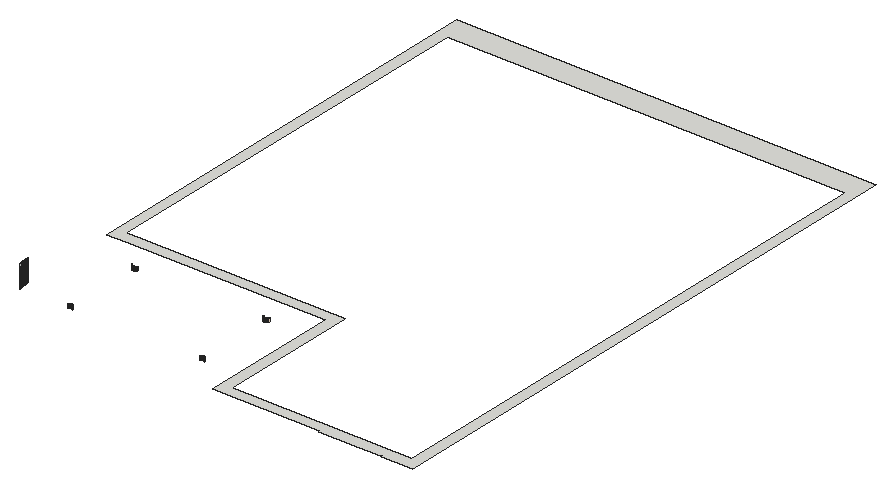
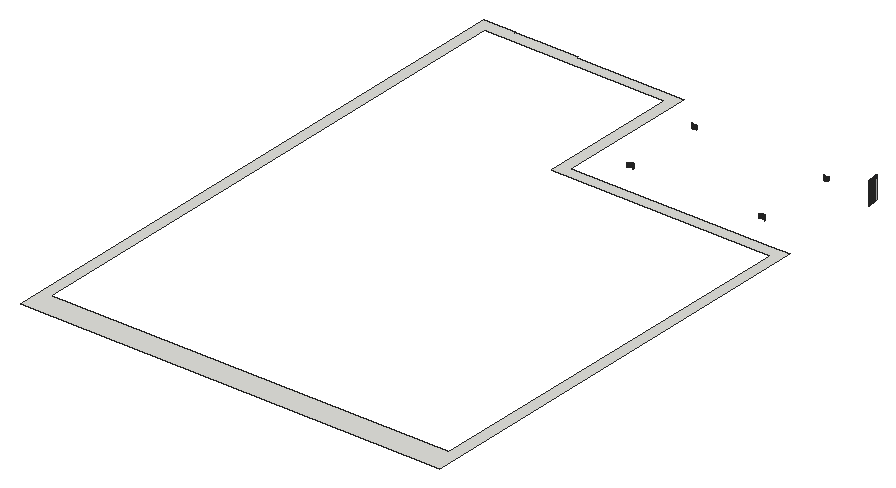
# SketchUp Ruby script. Lengths in inches.
U = 1.inch
M = Sketchup.active_model
def pt(a) = Geom::Point3d.new(a.map { |v| v * U })
def face(e, loops, mat)
  f = e.add_face(loops[0].map { |a| pt(a) })
  loops[1..].each { |l| e.add_face(l.map { |a| pt(a) }).erase! }
  f.material = f.back_material = mat if mat
  f
end
# faces: each face lists its corners as indices into pts; further lists are holes
def faces(e, pts, list, mat = nil) = list.each { |f| face(e, (f[0].is_a?(Array) ? f : [f]).map { |l| l.map { |i| pts[i] } }, mat) }
# xy, xz, yz: faces in a plane at the given z, y or x. An outline is a flat list of corners, or four numbers for a rectangle; further outlines are holes
def ring(l) = l.size == 4 ? [[l[0], l[1]], [l[2], l[1]], [l[2], l[3]], [l[0], l[3]]] : l.each_slice(2).to_a
def flat(e, list, mat, &to3) = list.each { |f| face(e, (f[0].is_a?(Array) ? f : [f]).map { |l| ring(l).map { |u, v| to3.(u, v) } }, mat) }
def xy(e, z, list, mat = nil) = flat(e, list, mat) { |x, y| [x, y, z] }
def xz(e, y, list, mat = nil) = flat(e, list, mat) { |x, z| [x, y, z] }
def yz(e, x, list, mat = nil) = flat(e, list, mat) { |y, z| [x, y, z] }
def lines(e, pts, list) = list.each { |a, b| e.add_line(pt(pts[a]), pt(pts[b])) }
# prism: a flat outline (further loops are holes) pulled along v
def prism(e, loops, v, mat = nil)
  f = face(e, loops, mat); d = Geom::Vector3d.new(v.map { |x| x * U })
  f.pushpull(f.normal.samedirection?(d) ? d.length : -d.length)
end
def box(e, o, s, mat = nil) = prism(e, [[o, [o[0] + s[0], o[1], o[2]], [o[0] + s[0], o[1] + s[1], o[2]], [o[0], o[1] + s[1], o[2]]]], [0, 0, s[2]], mat)
def at(x, y, z, deg = 0) = Geom::Transformation.translation(pt([x, y, z])) * Geom::Transformation.rotation(ORIGIN, Z_AXIS, deg.degrees)
def axes(o, x, y, z) = Geom::Transformation.new([*x, 0, *y, 0, *z, 0, *pt(o).to_a, 1])
def part(name) = M.definitions.add(name)
# library, detail: a bought-in or finely detailed component or shape, given as its bounding box
def library(name, o, s) = part(name).tap { |d| box(d.entities, o, s) }
def detail(e, o, s) = box(e.add_group.entities, o, s)
def put(e, d, t, mat = nil) = e.add_instance(d, t).tap { |i| i.material = mat if mat }
def group(e, t, mat = nil) = e.add_group.tap { |g| g.transformation = t; g.material = mat if mat }.entities
root = M.entities
M.materials.add("1122 AP 7994 PEACH ROSE").color = [254, 227, 201]
M.materials.add("[Quartz Light Grey]").color = [251, 251, 252]
xy(root,278.82,[[[286.125,152,320.75,152,320.75,153.25,321,153.25,321,152,338.75,152,338.75,153.25,339.75,153.25,339.75,152,366,152,366,645,9,645,9,273,25,273,25,273.25,25.25,273.25,25.25,273,195,273,195,153,286.125,153],[204,162,204,282,18,282,18,624,357,624,357,162]]])
xz(root,180,[[52.82,278.82,52.9,281.82],[52.9,278.82,52.98,281.82],[52.98,278.82,53.06,281.82],[53.06,278.82,53.14,281.82],[164.84,278.82,164.92,281.82],
  [164.92,278.82,165,281.82],[165,278.82,165.08,281.82],[165.08,278.82,165.16,281.82]],"1122 AP 7994 PEACH ROSE")
xz(root,246,[[52.82,278.82,52.9,281.82],[52.9,278.82,52.98,281.82],[52.98,278.82,53.06,281.82],[53.06,278.82,53.14,281.82],[164.84,278.82,164.92,281.82],
  [164.92,278.82,165,281.82],[165,278.82,165.08,281.82],[165.08,278.82,165.16,281.82]],"1122 AP 7994 PEACH ROSE")
yz(root,9,[[188.6875,278.82,189,297.82]],"[Quartz Light Grey]")
yz(root,9.01,[[188.06,278.82,188.37,297.82]],"[Quartz Light Grey]")
p = [[50.75,179.01,278.82],[50.8,179.07,278.82],[50.8,179.07,281.82],[50.75,179.01,281.82],[55.16,179.07,278.82],[55.21,179.01,278.82],
  [55.21,179.01,281.82],[55.16,179.07,281.82],[162.77,179.01,278.82],[162.82,179.07,278.82],[162.82,179.07,281.82],[162.77,179.01,281.82],
  [167.18,179.07,278.82],[167.23,179.01,278.82],[167.23,179.01,281.82],[167.18,179.07,281.82],[10.31,179.38,278.82],[10.39,179.08,278.82],
  [10.39,179.08,297.82],[10.31,179.38,297.82],[50.86,179.12,278.82],[50.86,179.12,281.82],[50.92,179.18,278.82],[50.92,179.18,281.82],
  [55.05,179.18,278.82],[55.1,179.12,278.82],[55.1,179.12,281.82],[55.05,179.18,281.82],[162.88,179.12,278.82],[162.88,179.12,281.82],
  [162.93,179.18,278.82],[162.93,179.18,281.82],[167.12,179.12,278.82],[167.12,179.12,281.82],[167.07,179.18,278.82],[167.07,179.18,281.82],
  [50.97,179.23,278.82],[50.97,179.23,281.82],[51.03,179.28,278.82],[51.03,179.28,281.82],[54.93,179.28,278.82],[54.99,179.23,278.82],
  [54.99,179.23,281.82],[54.93,179.28,281.82],[162.99,179.23,278.82],[162.99,179.23,281.82],[163.05,179.28,278.82],[163.05,179.28,281.82],
  [166.95,179.28,278.82],[167.01,179.23,278.82],[167.01,179.23,281.82],[166.95,179.28,281.82],[51.09,179.33,278.82],[51.09,179.33,281.82],
  [51.15,179.38,278.82],[51.15,179.38,281.82],[54.81,179.38,278.82],[54.87,179.33,278.82],[54.87,179.33,281.82],[54.81,179.38,281.82],
  [163.11,179.33,278.82],[163.11,179.33,281.82],[163.17,179.38,278.82],[163.17,179.38,281.82],[166.83,179.38,278.82],[166.89,179.33,278.82],
  [166.89,179.33,281.82],[166.83,179.38,281.82],[10.23,179.68,278.82],[10.23,179.68,297.82],[51.22,179.43,278.82],[51.22,179.43,281.82],
  [51.28,179.47,278.82],[51.28,179.47,281.82],[54.74,179.43,278.82],[54.74,179.43,281.82],[54.68,179.47,278.82],[54.68,179.47,281.82],
  [163.24,179.43,278.82],[163.24,179.43,281.82],[163.3,179.47,278.82],[163.3,179.47,281.82],[166.7,179.47,278.82],[166.76,179.43,278.82],
  [166.76,179.43,281.82],[166.7,179.47,281.82],[51.35,179.52,278.82],[51.35,179.52,281.82],[51.41,179.56,278.82],[51.41,179.56,281.82],
  [54.55,179.56,278.82],[54.61,179.52,278.82],[54.61,179.52,281.82],[54.55,179.56,281.82],[163.37,179.52,278.82],[163.37,179.52,281.82],
  [163.43,179.56,278.82],[163.43,179.56,281.82],[166.63,179.52,278.82],[166.63,179.52,281.82],[166.57,179.56,278.82],[166.57,179.56,281.82],
  [51.48,179.6,278.82],[51.48,179.6,281.82],[51.55,179.64,278.82],[51.55,179.64,281.82],[51.62,179.67,278.82],[51.62,179.67,281.82],
  [54.34,179.67,278.82],[54.41,179.64,278.82],[54.41,179.64,281.82],[54.34,179.67,281.82],[54.48,179.6,278.82],[54.48,179.6,281.82],
  [163.5,179.6,278.82],[163.5,179.6,281.82],[163.57,179.64,278.82],[163.57,179.64,281.82],[163.64,179.67,278.82],[163.64,179.67,281.82],
  [166.43,179.64,278.82],[166.5,179.6,278.82],[166.5,179.6,281.82],[166.43,179.64,281.82],[166.36,179.67,278.82],[166.36,179.67,281.82],
  [10.15,179.99,278.82],[10.15,179.99,297.82],[51.6875,179.71,278.82],[51.6875,179.71,281.82],[51.76,179.74,278.82],[51.76,179.74,281.82],
  [51.83,179.77,278.82],[51.83,179.77,281.82],[54.13,179.77,278.82],[54.2,179.74,278.82],[54.2,179.74,281.82],[54.13,179.77,281.82],
  [54.27,179.71,278.82],[54.27,179.71,281.82],[163.71,179.71,278.82],[163.71,179.71,281.82],[163.78,179.74,278.82],[163.78,179.74,281.82],
  [163.85,179.77,278.82],[163.85,179.77,281.82],[166.15,179.77,278.82],[166.22,179.74,278.82],[166.22,179.74,281.82],[166.15,179.77,281.82],
  [166.29,179.71,278.82],[166.29,179.71,281.82],[51.91,179.8,278.82],[51.91,179.8,281.82],[51.98,179.83,278.82],[51.98,179.83,281.82],
  [52.05,179.85,278.82],[52.05,179.85,281.82],[53.91,179.85,278.82],[53.98,179.83,278.82],[53.98,179.83,281.82],[53.91,179.85,281.82],
  [54.06,179.8,278.82],[54.06,179.8,281.82],[163.92,179.8,278.82],[163.92,179.8,281.82],[164,179.83,278.82],[164,179.83,281.82],
  [164.07,179.85,278.82],[164.07,179.85,281.82],[165.93,179.85,278.82],[166,179.83,278.82],[166,179.83,281.82],[165.93,179.85,281.82],
  [166.08,179.8,278.82],[166.08,179.8,281.82],[52.13,179.875,278.82],[52.13,179.875,281.82],[52.2,179.9,278.82],[52.2,179.9,281.82],
  [52.28,179.92,278.82],[52.28,179.92,281.82],[52.36,179.93,278.82],[52.36,179.93,281.82],[52.43,179.95,278.82],[52.43,179.95,281.82],
  [52.51,179.96,278.82],[52.51,179.96,281.82],[53.53,179.95,278.82],[53.6,179.93,278.82],[53.6,179.93,281.82],[53.53,179.95,281.82],
  [53.45,179.96,278.82],[53.45,179.96,281.82],[53.68,179.92,278.82],[53.68,179.92,281.82],[53.76,179.9,278.82],[53.76,179.9,281.82],
  [53.83,179.875,278.82],[53.83,179.875,281.82],[164.15,179.875,278.82],[164.15,179.875,281.82],[164.22,179.9,278.82],[164.22,179.9,281.82],
  [164.3,179.92,278.82],[164.3,179.92,281.82],[164.375,179.93,278.82],[164.375,179.93,281.82],[164.45,179.95,278.82],[164.45,179.95,281.82],
  [164.53,179.96,278.82],[164.53,179.96,281.82],[165.55,179.95,278.82],[165.625,179.93,278.82],[165.625,179.93,281.82],[165.55,179.95,281.82],
  [165.47,179.96,278.82],[165.47,179.96,281.82],[165.7,179.92,278.82],[165.7,179.92,281.82],[165.78,179.9,278.82],[165.78,179.9,281.82],
  [165.85,179.875,278.82],[165.85,179.875,281.82],[10.07,180.29,278.82],[10.07,180.29,297.82],[52.59,179.97,278.82],[52.59,179.97,281.82],
  [52.67,179.98,278.82],[52.67,179.98,281.82],[52.75,179.99,278.82],[52.75,179.99,281.82],[52.82,180,278.82],[52.82,180,281.82],
  [53.14,180,278.82],[53.22,179.99,278.82],[53.22,179.99,281.82],[53.14,180,281.82],[53.29,179.98,278.82],[53.29,179.98,281.82],
  [53.37,179.97,278.82],[53.37,179.97,281.82],[164.61,179.97,278.82],[164.61,179.97,281.82],[164.6875,179.98,278.82],[164.6875,179.98,281.82],
  [164.76,179.99,278.82],[164.76,179.99,281.82],[164.84,180,278.82],[164.84,180,281.82],[165.24,179.99,278.82],[165.3125,179.98,278.82],
  [165.3125,179.98,281.82],[165.24,179.99,281.82],[165.16,180,278.82],[165.16,180,281.82],[165.39,179.97,278.82],[165.39,179.97,281.82],
  [9.99,180.6,278.82],[9.99,180.6,297.82],[9.92,180.9,278.82],[9.92,180.9,297.82],[9.85,181.21,278.82],[9.85,181.21,297.82],
  [9.79,181.52,278.82],[9.79,181.52,297.82],[9.72,181.82,278.82],[9.72,181.82,297.82],[9.66,182.13,278.82],[9.66,182.13,297.82],
  [9.6,182.44,278.82],[9.6,182.44,297.82],[9.55,182.75,278.82],[9.55,182.75,297.82],[9.49,183.06,278.82],[9.49,183.06,297.82],
  [9.44,183.37,278.82],[9.44,183.37,297.82],[9.4,183.68,278.82],[9.4,183.68,297.82],[9.35,183.99,278.82],[9.35,183.99,297.82],
  [9.31,184.3,278.82],[9.31,184.3,297.82],[9.27,184.61,278.82],[9.27,184.61,297.82],[9.23,184.92,278.82],[9.23,184.92,297.82],
  [9.2,185.24,278.82],[9.2,185.24,297.82],[9.17,185.55,278.82],[9.17,185.55,297.82],[9.14,185.86,278.82],[9.14,185.86,297.82],
  [9.11,186.18,278.82],[9.11,186.18,297.82],[9.09,186.49,278.82],[9.09,186.49,297.82],[9.07,186.8,278.82],[9.07,186.8,297.82],
  [9.05,187.12,278.82],[9.05,187.12,297.82],[9.03,187.43,278.82],[9.03,187.43,297.82],[9.02,187.74,278.82],[9.02,187.74,297.82],
  [9.01,188.06,278.82],[9.01,188.06,297.82],[9,188.6875,278.82],[9.01,188.37,278.82],[9.01,188.37,297.82],[9,188.6875,297.82],
  [52.51,246.04,278.82],[52.43,246.05,278.82],[52.43,246.05,281.82],[52.51,246.04,281.82],[52.59,246.03,278.82],[52.59,246.03,281.82],
  [52.67,246.02,278.82],[52.67,246.02,281.82],[52.82,246,278.82],[52.75,246.01,278.82],[52.75,246.01,281.82],[52.82,246,281.82],
  [53.22,246.01,278.82],[53.14,246,278.82],[53.14,246,281.82],[53.22,246.01,281.82],[53.29,246.02,278.82],[53.29,246.02,281.82],
  [53.37,246.03,278.82],[53.37,246.03,281.82],[53.45,246.04,278.82],[53.45,246.04,281.82],[53.53,246.05,278.82],[53.53,246.05,281.82],
  [164.61,246.03,278.82],[164.53,246.04,278.82],[164.53,246.04,281.82],[164.61,246.03,281.82],[164.45,246.05,278.82],[164.45,246.05,281.82],
  [164.6875,246.02,278.82],[164.6875,246.02,281.82],[164.76,246.01,278.82],[164.76,246.01,281.82],[164.84,246,278.82],[164.84,246,281.82],
  [165.24,246.01,278.82],[165.16,246,278.82],[165.16,246,281.82],[165.24,246.01,281.82],[165.3125,246.02,278.82],[165.3125,246.02,281.82],
  [165.39,246.03,278.82],[165.39,246.03,281.82],[165.47,246.04,278.82],[165.47,246.04,281.82],[165.55,246.05,278.82],[165.55,246.05,281.82],
  [52.05,246.15,278.82],[51.98,246.17,278.82],[51.98,246.17,281.82],[52.05,246.15,281.82],[52.2,246.1,278.82],[52.13,246.125,278.82],
  [52.13,246.125,281.82],[52.2,246.1,281.82],[52.28,246.08,278.82],[52.28,246.08,281.82],[52.36,246.07,278.82],[52.36,246.07,281.82],
  [53.6,246.07,278.82],[53.6,246.07,281.82],[53.68,246.08,278.82],[53.68,246.08,281.82],[53.76,246.1,278.82],[53.76,246.1,281.82],
  [53.83,246.125,278.82],[53.83,246.125,281.82],[53.91,246.15,278.82],[53.91,246.15,281.82],[53.98,246.17,278.82],[53.98,246.17,281.82],
  [164.07,246.15,278.82],[164,246.17,278.82],[164,246.17,281.82],[164.07,246.15,281.82],[164.22,246.1,278.82],[164.15,246.125,278.82],
  [164.15,246.125,281.82],[164.22,246.1,281.82],[164.3,246.08,278.82],[164.3,246.08,281.82],[164.375,246.07,278.82],[164.375,246.07,281.82],
  [165.625,246.07,278.82],[165.625,246.07,281.82],[165.7,246.08,278.82],[165.7,246.08,281.82],[165.78,246.1,278.82],[165.78,246.1,281.82],
  [165.85,246.125,278.82],[165.85,246.125,281.82],[165.93,246.15,278.82],[165.93,246.15,281.82],[166,246.17,278.82],[166,246.17,281.82],
  [51.91,246.2,278.82],[51.83,246.23,278.82],[51.83,246.23,281.82],[51.91,246.2,281.82],[51.76,246.26,278.82],[51.76,246.26,281.82],
  [54.06,246.2,278.82],[54.06,246.2,281.82],[54.13,246.23,278.82],[54.13,246.23,281.82],[54.2,246.26,278.82],[54.2,246.26,281.82],
  [163.85,246.23,278.82],[163.78,246.26,278.82],[163.78,246.26,281.82],[163.85,246.23,281.82],[163.92,246.2,278.82],[163.92,246.2,281.82],
  [166.08,246.2,278.82],[166.08,246.2,281.82],[166.15,246.23,278.82],[166.15,246.23,281.82],[166.22,246.26,278.82],[166.22,246.26,281.82],
  [51.62,246.33,278.82],[51.55,246.36,278.82],[51.55,246.36,281.82],[51.62,246.33,281.82],[51.6875,246.29,278.82],[51.6875,246.29,281.82],
  [54.27,246.29,278.82],[54.27,246.29,281.82],[54.34,246.33,278.82],[54.34,246.33,281.82],[54.41,246.36,278.82],[54.41,246.36,281.82],
  [163.71,246.29,278.82],[163.64,246.33,278.82],[163.64,246.33,281.82],[163.71,246.29,281.82],[163.57,246.36,278.82],[163.57,246.36,281.82],
  [166.29,246.29,278.82],[166.29,246.29,281.82],[166.36,246.33,278.82],[166.36,246.33,281.82],[166.43,246.36,278.82],[166.43,246.36,281.82],
  [51.41,246.44,278.82],[51.35,246.48,278.82],[51.35,246.48,281.82],[51.41,246.44,281.82],[51.48,246.4,278.82],[51.48,246.4,281.82],
  [54.48,246.4,278.82],[54.48,246.4,281.82],[54.55,246.44,278.82],[54.55,246.44,281.82],[54.61,246.48,278.82],[54.61,246.48,281.82],
  [163.5,246.4,278.82],[163.43,246.44,278.82],[163.43,246.44,281.82],[163.5,246.4,281.82],[163.37,246.48,278.82],[163.37,246.48,281.82],
  [166.5,246.4,278.82],[166.5,246.4,281.82],[166.57,246.44,278.82],[166.57,246.44,281.82],[166.63,246.48,278.82],[166.63,246.48,281.82],
  [51.28,246.53,278.82],[51.22,246.57,278.82],[51.22,246.57,281.82],[51.28,246.53,281.82],[54.68,246.53,278.82],[54.68,246.53,281.82],
  [54.74,246.57,278.82],[54.74,246.57,281.82],[163.3,246.53,278.82],[163.24,246.57,278.82],[163.24,246.57,281.82],[163.3,246.53,281.82],
  [166.7,246.53,278.82],[166.7,246.53,281.82],[166.76,246.57,278.82],[166.76,246.57,281.82],[51.15,246.62,278.82],[51.09,246.67,278.82],
  [51.09,246.67,281.82],[51.15,246.62,281.82],[54.81,246.62,278.82],[54.81,246.62,281.82],[54.87,246.67,278.82],[54.87,246.67,281.82],
  [163.17,246.62,278.82],[163.11,246.67,278.82],[163.11,246.67,281.82],[163.17,246.62,281.82],[166.83,246.62,278.82],[166.83,246.62,281.82],
  [166.89,246.67,278.82],[166.89,246.67,281.82],[51.03,246.72,278.82],[51.03,246.72,281.82],[50.97,246.77,278.82],[50.97,246.77,281.82],
  [54.93,246.72,278.82],[54.93,246.72,281.82],[54.99,246.77,278.82],[54.99,246.77,281.82],[163.05,246.72,278.82],[162.99,246.77,278.82],
  [162.99,246.77,281.82],[163.05,246.72,281.82],[166.95,246.72,278.82],[166.95,246.72,281.82],[167.01,246.77,278.82],[167.01,246.77,281.82],
  [50.92,246.82,278.82],[50.92,246.82,281.82],[50.86,246.88,278.82],[50.86,246.88,281.82],[55.05,246.82,278.82],[55.05,246.82,281.82],
  [55.1,246.88,278.82],[55.1,246.88,281.82],[162.93,246.82,278.82],[162.93,246.82,281.82],[162.88,246.88,278.82],[162.88,246.88,281.82],
  [167.07,246.82,278.82],[167.07,246.82,281.82],[167.12,246.88,278.82],[167.12,246.88,281.82],[50.8,246.93,278.82],[50.8,246.93,281.82],
  [50.75,246.99,278.82],[50.75,246.99,281.82],[55.16,246.93,278.82],[55.16,246.93,281.82],[55.21,246.99,278.82],[55.21,246.99,281.82],
  [162.82,246.93,278.82],[162.82,246.93,281.82],[162.77,246.99,278.82],[162.77,246.99,281.82],[167.18,246.93,278.82],[167.18,246.93,281.82],
  [167.23,246.99,278.82],[167.23,246.99,281.82],[50.7,247.05,278.82],[50.7,247.05,281.82],[55.26,247.05,278.82],[55.26,247.05,281.82],
  [162.72,247.05,278.82],[162.72,247.05,281.82],[167.28,247.05,278.82],[167.28,247.05,281.82],[50.65,247.11,278.82],[50.65,247.11,281.82],
  [50.6,247.17,278.82],[50.6,247.17,281.82],[55.3125,247.11,278.82],[55.3125,247.11,281.82],[55.36,247.17,278.82],[55.36,247.17,281.82],
  [162.67,247.11,278.82],[162.62,247.17,278.82],[162.62,247.17,281.82],[162.67,247.11,281.82],[167.33,247.11,278.82],[167.33,247.11,281.82],
  [167.38,247.17,278.82],[167.38,247.17,281.82],[50.55,247.24,278.82],[50.51,247.3,278.82],[50.51,247.3,281.82],[50.55,247.24,281.82],
  [55.41,247.24,278.82],[55.41,247.24,281.82],[55.45,247.3,278.82],[55.45,247.3,281.82],[162.57,247.24,278.82],[162.53,247.3,278.82],
  [162.53,247.3,281.82],[162.57,247.24,281.82],[167.43,247.24,278.82],[167.43,247.24,281.82],[167.47,247.3,278.82],[167.47,247.3,281.82],
  [50.46,247.37,278.82],[50.46,247.37,281.82],[55.5,247.37,278.82],[55.5,247.37,281.82],[162.48,247.37,278.82],[162.48,247.37,281.82],
  [167.52,247.37,278.82],[167.52,247.37,281.82],[50.42,247.43,278.82],[50.42,247.43,281.82],[50.38,247.5,278.82],[50.38,247.5,281.82],
  [55.54,247.43,278.82],[55.54,247.43,281.82],[55.58,247.5,278.82],[55.58,247.5,281.82],[162.44,247.43,278.82],[162.44,247.43,281.82],
  [162.4,247.5,278.82],[162.4,247.5,281.82],[167.56,247.43,278.82],[167.56,247.43,281.82],[167.6,247.5,278.82],[167.6,247.5,281.82],
  [50.34,247.57,278.82],[50.34,247.57,281.82],[55.62,247.57,278.82],[55.62,247.57,281.82],[162.36,247.57,278.82],[162.36,247.57,281.82]]
faces(root,p,[[0,1,2,3],[4,5,6,7],[8,9,10,11],[12,13,14,15],[1,20,21,2],[20,22,23,21],[24,25,26,27],[25,4,7,26],
  [9,28,29,10],[28,30,31,29],[32,12,15,33],[34,32,33,35],[22,36,37,23],[36,38,39,37],[40,41,42,43],[41,24,27,42],
  [30,44,45,31],[44,46,47,45],[48,49,50,51],[49,34,35,50],[38,52,53,39],[52,54,55,53],[56,57,58,59],[57,40,43,58],
  [46,60,61,47],[60,62,63,61],[64,65,66,67],[65,48,51,66],[54,70,71,55],[70,72,73,71],[74,56,59,75],[76,74,75,77],
  [62,78,79,63],[78,80,81,79],[82,83,84,85],[83,64,67,84],[72,86,87,73],[86,88,89,87],[90,91,92,93],[91,76,77,92],
  [80,94,95,81],[94,96,97,95],[98,82,85,99],[100,98,99,101],[88,102,103,89],[102,104,105,103],[104,106,107,105],[108,109,110,111],
  [109,112,113,110],[112,90,93,113],[96,114,115,97],[114,116,117,115],[116,118,119,117],[120,121,122,123],[124,120,123,125],[121,100,101,122],
  [106,128,129,107],[128,130,131,129],[130,132,133,131],[134,135,136,137],[135,138,139,136],[138,108,111,139],[118,140,141,119],[140,142,143,141],
  [142,144,145,143],[146,147,148,149],[147,150,151,148],[150,124,125,151],[132,152,153,133],[152,154,155,153],[154,156,157,155],[158,159,160,161],
  [159,162,163,160],[162,134,137,163],[144,164,165,145],[164,166,167,165],[166,168,169,167],[170,171,172,173],[171,174,175,172],[174,146,149,175],
  [156,176,177,157],[176,178,179,177],[178,180,181,179],[180,182,183,181],[182,184,185,183],[184,186,187,185],[188,189,190,191],[192,188,191,193],
  [189,194,195,190],[194,196,197,195],[198,158,161,199],[196,198,199,197],[168,200,201,169],[200,202,203,201],[202,204,205,203],[204,206,207,205],
  [206,208,209,207],[208,210,211,209],[212,213,214,215],[216,212,215,217],[213,218,219,214],[218,220,221,219],[220,222,223,221],[222,170,173,223],
  [186,226,227,187],[226,228,229,227],[228,230,231,229],[230,232,233,231],[234,235,236,237],[235,238,239,236],[238,240,241,239],[240,192,193,241],
  [210,242,243,211],[242,244,245,243],[244,246,247,245],[246,248,249,247],[250,251,252,253],[254,250,253,255],[251,256,257,252],[256,216,217,257],
  [312,313,314,315],[316,312,315,317],[318,316,317,319],[320,321,322,323],[321,318,319,322],[324,325,326,327],[328,324,327,329],[330,328,329,331],
  [332,330,331,333],[334,332,333,335],[336,337,338,339],[337,340,341,338],[342,336,339,343],[344,342,343,345],[346,344,345,347],[348,349,350,351],
  [352,348,351,353],[354,352,353,355],[356,354,355,357],[358,356,357,359],[360,361,362,363],[364,365,366,367],[365,360,363,366],[368,364,367,369],
  [370,368,369,371],[313,370,371,314],[372,334,335,373],[374,372,373,375],[376,374,375,377],[378,376,377,379],[380,378,379,381],[382,380,381,383],
  [384,385,386,387],[388,389,390,391],[389,384,387,390],[392,388,391,393],[394,392,393,395],[340,394,395,341],[396,358,359,397],[398,396,397,399],
  [400,398,399,401],[402,400,401,403],[404,402,403,405],[406,404,405,407],[408,409,410,411],[409,412,413,410],[361,408,411,362],[414,382,383,415],
  [416,414,415,417],[418,416,417,419],[420,421,422,423],[385,424,425,386],[424,420,423,425],[426,406,407,427],[428,426,427,429],[430,428,429,431],
  [432,433,434,435],[436,432,435,437],[412,436,437,413],[438,418,419,439],[440,438,439,441],[442,440,441,443],[444,445,446,447],[445,448,449,446],
  [421,444,447,422],[450,430,431,451],[452,450,451,453],[454,452,453,455],[456,457,458,459],[460,456,459,461],[433,460,461,434],[462,442,443,463],
  [464,462,463,465],[466,464,465,467],[468,469,470,471],[469,472,473,470],[448,468,471,449],[474,454,455,475],[476,474,475,477],[478,476,477,479],
  [480,481,482,483],[457,480,483,458],[484,466,467,485],[486,484,485,487],[488,489,490,491],[472,488,491,473],[492,478,479,493],[494,492,493,495],
  [496,497,498,499],[481,496,499,482],[500,486,487,501],[502,500,501,503],[504,505,506,507],[489,504,507,490],[508,494,495,509],[510,508,509,511],
  [497,512,513,498],[512,514,515,513],[516,502,503,517],[518,516,517,519],[520,521,522,523],[505,520,523,506],[524,510,511,525],[526,524,525,527],
  [514,528,529,515],[528,530,531,529],[532,518,519,533],[534,532,533,535],[521,536,537,522],[536,538,539,537],[540,526,527,541],[542,540,541,543],
  [530,544,545,531],[544,546,547,545],[548,534,535,549],[550,548,549,551],[538,552,553,539],[552,554,555,553],[556,542,543,557],[558,556,557,559],
  [546,560,561,547],[562,550,551,563],[554,564,565,555],[566,558,559,567],[560,568,569,561],[568,570,571,569],[572,562,563,573],[574,572,573,575],
  [576,577,578,579],[564,576,579,565],[580,566,567,581],[582,580,581,583],[584,585,586,587],[570,584,587,571],[588,574,575,589],[590,588,589,591],
  [592,593,594,595],[577,592,595,578],[596,582,583,597],[598,596,597,599],[585,600,601,586],[602,590,591,603],[593,604,605,594],[606,598,599,607],
  [600,608,609,601],[608,610,611,609],[612,602,603,613],[614,612,613,615],[604,616,617,605],[616,618,619,617],[620,606,607,621],[622,620,621,623],
  [610,624,625,611],[626,614,615,627],[618,628,629,619]],"1122 AP 7994 PEACH ROSE")
faces(root,p,[[16,17,18,19],[68,16,19,69],[126,68,69,127],[224,126,127,225],[258,224,225,259],[260,258,259,261],[262,260,261,263],[264,262,263,265],
  [266,264,265,267],[268,266,267,269],[270,268,269,271],[272,270,271,273],[274,272,273,275],[276,274,275,277],[278,276,277,279],[280,278,279,281],
  [282,280,281,283],[284,282,283,285],[286,284,285,287],[288,286,287,289],[290,288,289,291],[292,290,291,293],[294,292,293,295],[296,294,295,297],
  [298,296,297,299],[300,298,299,301],[302,300,301,303],[304,302,303,305],[306,304,305,307],[308,309,310,311]],"[Quartz Light Grey]")
